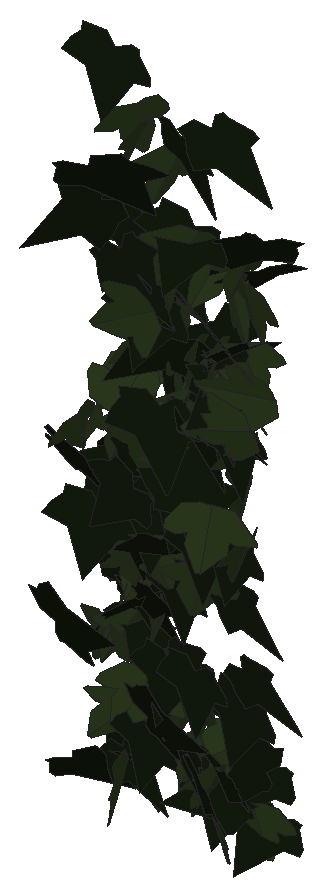
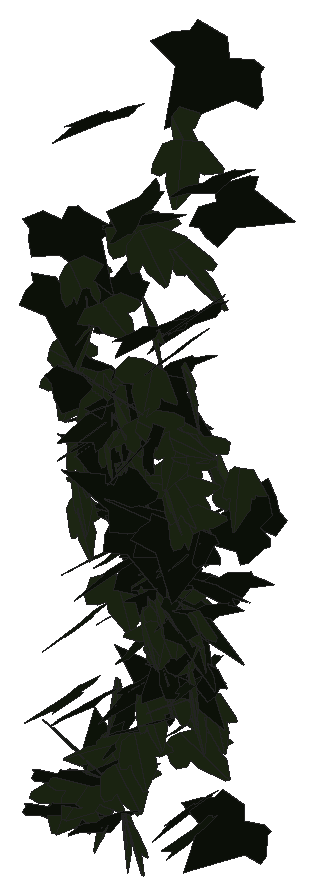
# SketchUp Ruby script. Lengths in inches.
U = 1.inch
M = Sketchup.active_model
def pt(a) = Geom::Point3d.new(a.map { |v| v * U })
def face(e, loops, mat)
  f = e.add_face(loops[0].map { |a| pt(a) })
  loops[1..].each { |l| e.add_face(l.map { |a| pt(a) }).erase! }
  f.material = f.back_material = mat if mat
  f
end
# faces: each face lists its corners as indices into pts; further lists are holes
def faces(e, pts, list, mat = nil) = list.each { |f| face(e, (f[0].is_a?(Array) ? f : [f]).map { |l| l.map { |i| pts[i] } }, mat) }
# xy, xz, yz: faces in a plane at the given z, y or x. An outline is a flat list of corners, or four numbers for a rectangle; further outlines are holes
def ring(l) = l.size == 4 ? [[l[0], l[1]], [l[2], l[1]], [l[2], l[3]], [l[0], l[3]]] : l.each_slice(2).to_a
def flat(e, list, mat, &to3) = list.each { |f| face(e, (f[0].is_a?(Array) ? f : [f]).map { |l| ring(l).map { |u, v| to3.(u, v) } }, mat) }
def xy(e, z, list, mat = nil) = flat(e, list, mat) { |x, y| [x, y, z] }
def xz(e, y, list, mat = nil) = flat(e, list, mat) { |x, z| [x, y, z] }
def yz(e, x, list, mat = nil) = flat(e, list, mat) { |y, z| [x, y, z] }
def lines(e, pts, list) = list.each { |a, b| e.add_line(pt(pts[a]), pt(pts[b])) }
# prism: a flat outline (further loops are holes) pulled along v
def prism(e, loops, v, mat = nil)
  f = face(e, loops, mat); d = Geom::Vector3d.new(v.map { |x| x * U })
  f.pushpull(f.normal.samedirection?(d) ? d.length : -d.length)
end
def box(e, o, s, mat = nil) = prism(e, [[o, [o[0] + s[0], o[1], o[2]], [o[0] + s[0], o[1] + s[1], o[2]], [o[0], o[1] + s[1], o[2]]]], [0, 0, s[2]], mat)
def at(x, y, z, deg = 0) = Geom::Transformation.translation(pt([x, y, z])) * Geom::Transformation.rotation(ORIGIN, Z_AXIS, deg.degrees)
def axes(o, x, y, z) = Geom::Transformation.new([*x, 0, *y, 0, *z, 0, *pt(o).to_a, 1])
def part(name) = M.definitions.add(name)
# library, detail: a bought-in or finely detailed component or shape, given as its bounding box
def library(name, o, s) = part(name).tap { |d| box(d.entities, o, s) }
def detail(e, o, s) = box(e.add_group.entities, o, s)
def put(e, d, t, mat = nil) = e.add_instance(d, t).tap { |i| i.material = mat if mat }
def group(e, t, mat = nil) = e.add_group.tap { |g| g.transformation = t; g.material = mat if mat }.entities
root = M.entities
M.materials.add("1026 AP 7946 SUNNY SIDE UP").color = [254, 231, 186]
M.materials.add("efeu1").color = [18, 25, 13]
M.materials.add("efeu2").color = [43, 57, 29]
c1 = part("ivyleaf_10")
p = [[0,0.5,-0.03],[-0.0625,2.02,-0.43],[-0.19,2.01,-0.46],[-0.54,1.05,-0.29],[-0.52,0.625,-0.18],[-0.83,0.76,-0.28],
  [-1.16,0.64,-0.33],[-1.15,0.33,-0.24],[-0.77,-0.39,0.02],[-0.3,-0.51,0.16],[0.04,-0.48,0.23],[-0.02,2.01,-0.4375],
  [-0.06,2.01,-0.43],[0.04,-0.49,0.23],[0.67,-0.49,0.14],[1.38,0.36,-0.2],[1.375,0.51,-0.24],[0.81,0.65,-0.19],
  [0.62,0.59,-0.15],[0.6,1.09,-0.28],[0.5,1.23,-0.31]]
faces(c1.entities,p,[[0,1,2,3,4,5,6,7,8,9,10],[11,12,0,13,14,15,16,17,18,19,20]],"efeu2")
c2 = part("ivyleaf_9")
p = [[1.54,2.16,1.25],[1.36,2.04,1.19],[-0.21,0.99,0.68],[-0.71,1.11,0.82],[-0.85,0.86,0.67],[-0.8,0.17,0.21],
  [-0.9,-0.01,0.1],[-0.67,-0.16,-0.02],[-0.08,-0.08,-0.05],[-0.03,-0.6,-0.4],[0.65,-0.88,-0.66],[0.83,-0.6,-0.49],
  [1.29,-0.42,-0.43],[1.8125,-0.07,-0.26],[1.21,0.44,0.15]]
faces(c2.entities,p,[[0,1,2,3,4,5,6,7,8,9,10,11,12,13,14]],"efeu1")
put(root,c1,axes([110.04,212.36,281.81],[-0.41666,0.10734,0.14692],[-0.23087,0.01217,-0.29167],[-0.15825,-0.30039,0.0387]),"1026 AP 7946 SUNNY SIDE UP")
put(root,c2,axes([109.94,212.88,284.09],[-0.47214,-0.12626,-0.0508],[0.11412,-0.05049,-0.32712],[0.17953,-0.29995,0.07433]),"1026 AP 7946 SUNNY SIDE UP")
put(root,c1,axes([109.9,211.86,285.31],[-0.0792,-0.30831,-0.14412],[0.04397,0.13539,-0.321],[0.52941,-0.05737,0.0051]),"1026 AP 7946 SUNNY SIDE UP")
put(root,c2,axes([109.79,212.8125,290.68],[-0.17446,-0.33344,0.05781],[0.00749,-0.06258,-0.36155],[0.53213,-0.10844,0.02404]),"1026 AP 7946 SUNNY SIDE UP")
put(root,c2,axes([109.52,211.96,284.73],[0.47639,-0.18609,0.10813],[0.1178,-0.07997,-0.36564],[0.31548,0.31086,-0.02674]),"1026 AP 7946 SUNNY SIDE UP")
put(root,c2,axes([109.76,212.02,279.81],[0.40702,0.22041,0.08662],[0.11869,0.03893,-0.34948],[-0.35069,0.26898,-0.01774]),"1026 AP 7946 SUNNY SIDE UP")
put(root,c2,axes([110.2,212.86,283.61],[-0.32806,0.22636,-0.11711],[0.00301,-0.14739,-0.30342],[-0.39919,-0.18714,0.09395]),"1026 AP 7946 SUNNY SIDE UP")
put(root,c1,axes([109.91,212.86,283.06],[-0.15896,0.28142,-0.13311],[0.00088,-0.13741,-0.30579],[-0.48797,-0.09192,0.04281]),"1026 AP 7946 SUNNY SIDE UP")
put(root,c1,axes([110.04,212.81,282.52],[0.1984,-0.29601,-0.13587],[-0.0281,0.13317,-0.32895],[0.50771,0.12305,0.03489]),"1026 AP 7946 SUNNY SIDE UP")
put(root,c2,axes([109.77,212.93,282.61],[0.17851,-0.30152,0.00504],[0.0021,-0.00656,-0.33195],[0.47422,0.11353,-0.00043]),"1026 AP 7946 SUNNY SIDE UP")
put(root,c2,axes([110.2,212.76,283.33],[-0.1289,0.31552,-0.02923],[0.0045,-0.03042,-0.33598],[-0.49837,-0.08188,0.00453]),"1026 AP 7946 SUNNY SIDE UP")
put(root,c1,axes([110.04,212.71,281.92],[0.11298,-0.31237,-0.0527],[0.0003,0.05068,-0.3297],[0.49726,0.07094,0.01218]),"1026 AP 7946 SUNNY SIDE UP")
put(root,c1,axes([110.1,212.8,284.97],[-0.16419,-0.30071,0.1012],[-0.01401,-0.1024,-0.3276],[0.49807,-0.10201,0.02414]),"1026 AP 7946 SUNNY SIDE UP")
put(root,c2,axes([109.92,212.86,283.61],[-0.18322,-0.30247,-0.04321],[0.05939,0.02843,-0.33278],[0.47611,-0.11995,0.02488]),"1026 AP 7946 SUNNY SIDE UP")
put(root,c1,axes([110.12,212.78,287.3],[0.23305,-0.29479,-0.1054],[-0.04314,0.09866,-0.33878],[0.4879,0.14953,0.02039]),"1026 AP 7946 SUNNY SIDE UP")
put(root,c2,axes([110.04,212.16,283.79],[-0.29842,-0.26578,-0.04943],[0.05476,0.03221,-0.33611],[0.4207,-0.19272,0.00869]),"1026 AP 7946 SUNNY SIDE UP")
put(root,c1,axes([110.05,212.02,285.23],[0.25096,-0.30946,0.13961],[-0.07581,0.12945,0.35912],[-0.5269,-0.16602,0.01483]),"1026 AP 7946 SUNNY SIDE UP")
put(root,c1,axes([110.21,212.8,285.4],[-0.15197,-0.28651,0.14751],[-0.01866,-0.14794,-0.31056],[0.50445,-0.09179,0.03295]),"1026 AP 7946 SUNNY SIDE UP")
put(root,c1,axes([110.19,212.92,283.47],[-0.51219,-0.0183,0.00928],[-0.01117,-0.03499,-0.33442],[0.03014,-0.32398,0.03367]),"1026 AP 7946 SUNNY SIDE UP")
put(root,c1,axes([110.1,212.8,282.99],[-0.42669,0.15548,-0.0781],[0.07139,-0.07375,-0.31994],[-0.26309,-0.27218,0.03985]),"1026 AP 7946 SUNNY SIDE UP")
put(root,c2,axes([110.17,212.84,284.76],[0.25049,0.28661,-0.04984],[-0.01719,-0.05107,-0.33775],[-0.45715,0.15897,-0.01461]),"1026 AP 7946 SUNNY SIDE UP")
put(root,c2,axes([109.81,212.88,282.82],[-0.03357,-0.03606,-0.33211],[0.48366,0.09971,-0.03191],[0.16098,-0.3071,0.02663]),"1026 AP 7946 SUNNY SIDE UP")
put(root,c1,axes([110.26,212.55,281.96],[-0.11931,-0.26401,0.18239],[-0.0022,-0.18325,-0.28084],[0.50114,-0.06366,0.04219]),"1026 AP 7946 SUNNY SIDE UP")
put(root,c2,axes([110.01,212.79,279.85],[0.1687,-0.29382,0.00052],[0.00743,-0.00059,-0.32221],[0.46196,0.10731,0.00499]),"1026 AP 7946 SUNNY SIDE UP")
put(root,c1,axes([110.62,212.93,286.4],[0.12624,-0.03617,-0.33517],[-0.50533,0.05388,-0.08761],[0.09619,0.33054,-0.02039]),"1026 AP 7946 SUNNY SIDE UP")
put(root,c1,axes([110.22,212.875,283.46],[-0.46451,0.1121,-0.0857],[0.07479,-0.10372,-0.31619],[-0.207,-0.28903,0.07807]),"1026 AP 7946 SUNNY SIDE UP")
put(root,c1,axes([110.1875,212.74,285.9],[0.31011,0.26192,-0.06047],[-0.02993,-0.06085,-0.33743],[-0.42151,0.19702,-0.02053]),"1026 AP 7946 SUNNY SIDE UP")
put(root,c2,axes([110.46,212.49,282.34],[-0.12383,0.26762,-0.16676],[-0.00197,-0.16874,-0.28508],[-0.49303,-0.06654,0.04302]),"1026 AP 7946 SUNNY SIDE UP")
put(root,c1,axes([110.33,212.87,283.67],[-0.11266,-0.30785,0.09073],[0.00004,-0.09203,-0.3255],[0.50424,-0.06877,0.0203]),"1026 AP 7946 SUNNY SIDE UP")
put(root,c1,axes([110.26,212.82,286.22],[-0.17743,-0.2893,-0.1302],[0.10691,0.10701,-0.31842],[0.48371,-0.12977,0.02262]),"1026 AP 7946 SUNNY SIDE UP")
put(root,c2,axes([110.12,212.59,288.3125],[0.09405,-0.34295,-0.02835],[0.00204,0.02618,-0.35843],[0.54075,0.05955,0.00628]),"1026 AP 7946 SUNNY SIDE UP")
put(root,c1,axes([110.4,212.92,283.68],[0.02679,-0.30085,0.12778],[0.01035,-0.12557,-0.31116],[0.51261,0.01826,-0.0004]),"1026 AP 7946 SUNNY SIDE UP")
put(root,c2,axes([110.11,212.85,284.5],[0.2487,-0.28915,-0.0526],[0.00641,0.05831,-0.33767],[0.46122,0.15511,0.03306]),"1026 AP 7946 SUNNY SIDE UP")
put(root,c1,axes([110.41,212.84,285.5],[0.11571,-0.3282,-0.03082],[-0.01063,0.02723,-0.34635],[0.51784,0.07389,-0.00022]),"1026 AP 7946 SUNNY SIDE UP")
put(root,c1,axes([110.46,212.8,282.91],[-0.30233,-0.20081,0.16911],[-0.01131,-0.20138,-0.26182],[0.40881,-0.15407,0.11782]),"1026 AP 7946 SUNNY SIDE UP")
put(root,c1,axes([110.59,212.16,280.88],[-0.33477,-0.11795,0.21363],[-0.19297,-0.18518,-0.23863],[0.32275,-0.23306,0.07892]),"1026 AP 7946 SUNNY SIDE UP")
put(root,c2,axes([110.09,212.68,284.8125],[0.50903,0.02201,0.07735],[0.11601,0.01895,-0.33387],[-0.0404,0.33175,0.01589]),"1026 AP 7946 SUNNY SIDE UP")
put(root,c2,axes([110.23,212.875,283.61],[0.22883,-0.28573,-0.0673],[-0.07302,0.04771,-0.32946],[0.45448,0.15153,-0.01905]),"1026 AP 7946 SUNNY SIDE UP")
put(root,c2,axes([110.45,212.82,281.85],[-0.19306,-0.2678,0.12855],[0.02907,-0.1434,-0.29555],[0.46466,-0.1023,0.0719]),"1026 AP 7946 SUNNY SIDE UP")
put(root,c1,axes([110.44,212.88,283.1],[0.29975,0.26211,0.03925],[-0.00229,0.04616,-0.33236],[-0.41615,0.18854,0.0301]),"1026 AP 7946 SUNNY SIDE UP")
put(root,c2,axes([110.36,212.35,280.02],[0.1753,-0.25838,-0.14486],[-0.05545,0.13598,-0.28843],[0.4581,0.11533,0.02052]),"1026 AP 7946 SUNNY SIDE UP")
put(root,c1,axes([110.61,212.32,283.28],[-0.17129,-0.30335,-0.03779],[0.0265,0.03109,-0.33182],[0.47942,-0.1101,0.00484]),"1026 AP 7946 SUNNY SIDE UP")
put(root,c2,axes([110.4,212.53,282.5],[0.49764,-0.03435,-0.06061],[-0.09767,-0.03285,-0.32571],[0.04336,0.32019,-0.038]),"1026 AP 7946 SUNNY SIDE UP")
put(root,c2,axes([110.47,212.73,287.57],[-0.05599,-0.31485,0.14173],[-0.02965,-0.13811,-0.32722],[0.54059,-0.04018,-0.00327]),"1026 AP 7946 SUNNY SIDE UP")
put(root,c1,axes([110.66,212.43,284.99],[-0.52543,0.01637,0.01731],[-0.02862,-0.03164,-0.34322],[-0.0231,-0.33308,0.03149]),"1026 AP 7946 SUNNY SIDE UP")
put(root,c2,axes([110.77,211.24,289.31],[-0.05967,-0.02786,-0.39694],[0.10582,-0.38156,0.01937],[-0.5979,-0.06475,0.04304]),"1026 AP 7946 SUNNY SIDE UP")
put(root,c2,axes([110.54,212.69,283.85],[-0.17492,-0.30837,-0.03718],[0.04587,0.02592,-0.33703],[0.48572,-0.1135,0.01844]),"1026 AP 7946 SUNNY SIDE UP")
put(root,c2,axes([110.46,212.87,283.74],[-0.05275,-0.30804,-0.11488],[0.08443,0.10366,-0.31598],[0.50722,-0.04929,0.04065]),"1026 AP 7946 SUNNY SIDE UP")
put(root,c2,axes([110.69,212.06,284.39],[-0.22147,-0.2116,0.21977],[-0.0842,-0.21547,-0.25642],[0.46627,-0.13942,0.05809]),"1026 AP 7946 SUNNY SIDE UP")
put(root,c1,axes([110.72,212.95,283.2],[0.07818,-0.31666,-0.04946],[-0.00094,0.04667,-0.32988],[0.5032,0.04929,0.00707]),"1026 AP 7946 SUNNY SIDE UP")
put(root,c2,axes([110.85,212.88,285.98],[0.01886,-0.12095,0.32264],[-0.04553,0.31253,0.12703],[-0.52694,-0.03134,0.00057]),"1026 AP 7946 SUNNY SIDE UP")
put(root,c2,axes([110.47,212.17,288],[0.1312,-0.29596,-0.19423],[-0.02416,0.18881,-0.31405],[0.54984,0.07892,0.03255]),"1026 AP 7946 SUNNY SIDE UP")
put(root,c1,axes([110.54,212.0625,285.73],[0.505,0.12235,-0.16015],[0.16605,0.1461,0.34254],[0.26405,-0.32586,0.09089]),"1026 AP 7946 SUNNY SIDE UP")
put(root,c1,axes([110.8,212.55,282.24],[0.17532,-0.2647,-0.15298],[-0.08397,0.137,-0.29507],[0.46862,0.12358,0.00436]),"1026 AP 7946 SUNNY SIDE UP")
put(root,c1,axes([110.61,212.95,283.48],[0.42521,-0.15269,0.09682],[0.11307,-0.06515,-0.31961],[0.25904,0.27907,-0.01943]),"1026 AP 7946 SUNNY SIDE UP")
put(root,c1,axes([110.79,212.87,287.19],[-0.5112,0.09624,0.01092],[-0.02827,-0.02546,-0.34811],[-0.1495,-0.32426,0.0285]),"1026 AP 7946 SUNNY SIDE UP")
put(root,c1,axes([110.83,212.84,289.32],[-0.17502,-0.31063,0.11971],[-0.00115,-0.12418,-0.3383],[0.52246,-0.10433,0.03936]),"1026 AP 7946 SUNNY SIDE UP")
put(root,c2,axes([110.93,212.86,284.63],[0.06964,0.29132,-0.15645],[-0.02346,-0.15297,-0.30436],[-0.51725,0.04616,-0.00726]),"1026 AP 7946 SUNNY SIDE UP")
put(root,c1,axes([110.83,212.03,290.43],[-0.25565,-0.33335,-0.08787],[0.07636,0.06905,-0.38144],[0.53489,-0.16918,0.01246]),"1026 AP 7946 SUNNY SIDE UP")
put(root,c2,axes([110.77,212.49,287.14],[-0.21482,-0.30826,0.07268],[-0.01923,-0.07354,-0.34728],[0.49749,-0.13595,0.01796]),"1026 AP 7946 SUNNY SIDE UP")
put(root,c1,axes([110.81,212.35,283.42],[-0.44558,-0.14871,-0.08246],[0.14181,-0.00298,-0.32668],[0.22377,-0.29422,0.04282]),"1026 AP 7946 SUNNY SIDE UP")
put(root,c1,axes([110.92,212.68,281.61],[-0.02839,-0.32295,0.02154],[0.00029,-0.02279,-0.33335],[0.50907,-0.018,0.00139]),"1026 AP 7946 SUNNY SIDE UP")
put(root,c2,axes([111.11,212.49,286.68],[0.02936,0.09354,-0.34254],[-0.12491,-0.32345,-0.10007],[-0.52939,0.08151,0.00461]),"1026 AP 7946 SUNNY SIDE UP")
put(root,c2,axes([111.06,212.26,283.61],[0.17392,0.28189,-0.15822],[-0.07174,-0.1487,-0.31264],[-0.50087,0.11918,-0.01016]),"1026 AP 7946 SUNNY SIDE UP")
put(root,c1,axes([111,211.98,281.47],[0.52597,0.0736,-0.11388],[-0.15666,-0.0607,-0.35124],[-0.13891,0.34716,-0.03508]),"1026 AP 7946 SUNNY SIDE UP")
put(root,c2,axes([110.75,212.75,287.92],[0.04706,-0.31716,-0.14479],[0.05467,0.14132,-0.32423],[0.54159,0.0133,0.04531]),"1026 AP 7946 SUNNY SIDE UP")
put(root,c1,axes([111.01,212.96,279.65],[0.30283,-0.23732,-0.04399],[-0.00947,0.04819,-0.31349],[0.37866,0.191,0.02734]),"1026 AP 7946 SUNNY SIDE UP")
put(root,c2,axes([110.98,213,284.97],[-0.38679,-0.19645,-0.10247],[0.16895,0.02121,-0.32036],[0.30131,-0.26407,0.04809]),"1026 AP 7946 SUNNY SIDE UP")
put(root,c2,axes([110.87,212.9,285.99],[0.20658,-0.29115,-0.11068],[-0.10296,0.08621,-0.3277],[0.47608,0.14498,-0.02284]),"1026 AP 7946 SUNNY SIDE UP")
put(root,c1,axes([111.02,212.84,286.29],[0.07666,0.31882,-0.10109],[-0.05894,-0.09514,-0.33207],[-0.52204,0.05756,0.02265]),"1026 AP 7946 SUNNY SIDE UP")
put(root,c2,axes([111.01,212.94,281.33],[-0.22303,-0.26383,0.10753],[0.01523,-0.12274,-0.30244],[0.44675,-0.12753,0.06399]),"1026 AP 7946 SUNNY SIDE UP")
put(root,c1,axes([111.12,212.68,280.89],[-0.14606,-0.30173,0.00557],[0.01114,-0.00963,-0.32514],[0.47444,-0.09266,0.00935]),"1026 AP 7946 SUNNY SIDE UP")
put(root,c2,axes([110.92,212.82,282.67],[-0.00412,-0.29575,0.13411],[0.02551,-0.13182,-0.30503],[0.50853,0.00422,0.01639]),"1026 AP 7946 SUNNY SIDE UP")
put(root,c1,axes([111.16,212.92,279.67],[0.13285,-0.27646,-0.11543],[0.00095,0.115,-0.29531],[0.46813,0.07822,0.03336]),"1026 AP 7946 SUNNY SIDE UP")
put(root,c1,axes([111.18,212.35,287.8],[0.29125,-0.28309,-0.08825],[-0.03686,0.08481,-0.34699],[0.46287,0.18488,0.02789]),"1026 AP 7946 SUNNY SIDE UP")
put(root,c2,axes([110.97,212.8,284.96],[0.15429,0.29054,-0.13288],[0.05794,0.12542,0.31661],[0.49753,-0.10471,0.00434]),"1026 AP 7946 SUNNY SIDE UP")
put(root,c2,axes([111.13,211.92,280.74],[-0.08525,-0.29,0.14491],[-0.0065,-0.14366,-0.30407],[0.5079,-0.05051,0.02043]),"1026 AP 7946 SUNNY SIDE UP")
put(root,c1,axes([111.26,211.54,290.49],[0.12831,-0.33596,0.10108],[0.03,-0.09829,-0.35672],[0.55037,0.08368,-0.00412]),"1026 AP 7946 SUNNY SIDE UP")
put(root,c1,axes([111.37,212.33,285.02],[-0.20512,-0.28387,0.11099],[-0.03528,-0.10968,-0.32153],[0.47703,-0.13018,0.02394]),"1026 AP 7946 SUNNY SIDE UP")
put(root,c1,axes([111.3125,212.28,281.375],[0.06316,-0.30272,0.09418],[0.02887,-0.0915,-0.31507],[0.49718,0.04377,0.00633]),"1026 AP 7946 SUNNY SIDE UP")
put(root,c2,axes([111.02,212.78,289.69],[0.18683,-0.32958,0.13084],[0.05591,-0.12414,-0.36156],[0.55364,0.12376,-0.00764]),"1026 AP 7946 SUNNY SIDE UP")
put(root,c2,axes([111.17,212.09,285.8],[-0.16122,-0.36141,-0.0643],[0.0645,0.05096,-0.38584],[0.57252,-0.10751,0.02537]),"1026 AP 7946 SUNNY SIDE UP")
put(root,c1,axes([111.4,212.72,280.3125],[-0.22353,-0.25621,0.11746],[-0.01996,-0.12342,-0.29893],[0.44144,-0.13531,0.04596]),"1026 AP 7946 SUNNY SIDE UP")
put(root,c1,axes([111.28,212.87,286.51],[0.13537,-0.29309,0.14519],[0.09749,-0.13008,-0.31474],[0.50316,0.10405,0.02192]),"1026 AP 7946 SUNNY SIDE UP")
put(root,c1,axes([111.44,212.65,285.77],[-0.27411,-0.26224,0.11837],[-0.02814,-0.12599,-0.32078],[0.45026,-0.16752,0.05202]),"1026 AP 7946 SUNNY SIDE UP")
put(root,c2,axes([111.35,212.52,284.48],[-0.42264,-0.15014,-0.13133],[0.1877,0.04555,-0.31642],[0.24524,-0.29361,0.01586]),"1026 AP 7946 SUNNY SIDE UP")
put(root,c2,axes([111.17,212.33,281.76],[0.1457,-0.2171,-0.23601],[-0.04767,0.23027,-0.23738],[0.49258,0.0865,0.04684]),"1026 AP 7946 SUNNY SIDE UP")
put(root,c2,axes([111.28,212.17,281.72],[-0.10456,-0.2876,0.13693],[-0.02091,-0.13482,-0.30445],[0.49883,-0.06593,0.01594]),"1026 AP 7946 SUNNY SIDE UP")
put(root,c1,axes([111.42,212.76,286.125],[0.09943,-0.3349,-0.01855],[0.03058,0.02002,-0.3502],[0.52632,0.0621,0.02385]),"1026 AP 7946 SUNNY SIDE UP")
put(root,c1,axes([111.72,210.95,288.02],[0.37388,-0.14777,-0.28081],[-0.37353,0.13228,-0.28747],[0.31151,0.33598,-0.00767]),"1026 AP 7946 SUNNY SIDE UP")
put(root,c2,axes([111.06,209.99,283.33],[0.07703,-0.08837,0.39051],[0.32588,-0.31807,-0.10571],[0.51897,0.21285,0.00841]),"1026 AP 7946 SUNNY SIDE UP")
put(root,c2,axes([111.27,212.66,283.89],[0.23626,-0.21641,-0.21497],[-0.07322,0.21238,-0.26175],[0.46564,0.1432,0.06791]),"1026 AP 7946 SUNNY SIDE UP")
put(root,c1,axes([111.56,212.69,285.62],[0.06744,-0.33524,0.0203],[0.004,-0.02146,-0.3483],[0.52821,0.04297,0.00004]),"1026 AP 7946 SUNNY SIDE UP")
put(root,c1,axes([111.37,210.98,280.65],[0.16006,-0.19305,0.32232],[0.26132,-0.26669,-0.226],[0.51729,0.19446,0.01444]),"1026 AP 7946 SUNNY SIDE UP")
put(root,c2,axes([111.94,212.875,286.78],[-0.36911,0.20931,0.13194],[-0.24318,0.00942,-0.31073],[-0.29831,-0.26667,0.09005]),"1026 AP 7946 SUNNY SIDE UP")
put(root,c1,axes([111.61,212.79,287.95],[0.26706,0.24758,-0.16732],[-0.1788,-0.12009,-0.30912],[-0.43121,0.20313,0.02455]),"1026 AP 7946 SUNNY SIDE UP")
put(root,c1,axes([111.7,212.43,283.19],[-0.44566,-0.14546,0.07633],[-0.07782,-0.06662,-0.32651],[0.24522,-0.28549,0.0351]),"1026 AP 7946 SUNNY SIDE UP")
put(root,c2,axes([111.39,212.55,285.57],[0.19152,-0.3133,0.05267],[0.00817,-0.05469,-0.34628],[0.49955,0.12101,-0.01453]),"1026 AP 7946 SUNNY SIDE UP")
put(root,c2,axes([111.42,212.21,280.66],[0.14807,-0.28591,0.12843],[0.02948,-0.12649,-0.31016],[0.49058,0.0939,-0.02012]),"1026 AP 7946 SUNNY SIDE UP")
put(root,c2,axes([111.62,212.97,279.59],[-0.16265,-0.28629,0.04824],[0.00135,-0.05174,-0.31334],[0.45656,-0.10184,0.01811]),"1026 AP 7946 SUNNY SIDE UP")
put(root,c2,axes([111.3,211.72,281.13],[0.14973,-0.11356,0.35167],[0.28627,-0.29012,-0.15316],[0.48901,0.20461,-0.01802]),"1026 AP 7946 SUNNY SIDE UP")
put(root,c2,axes([111.45,212.93,286.29],[0.39825,-0.2232,-0.00703],[-0.02958,-0.01296,-0.34711],[0.34982,0.253,-0.02135]),"1026 AP 7946 SUNNY SIDE UP")
put(root,c1,axes([111.88,211.88,288.81],[-0.27488,-0.2895,0.17147],[-0.08481,-0.16279,-0.34758],[0.5195,-0.17976,0.03399]),"1026 AP 7946 SUNNY SIDE UP")
put(root,c2,axes([111.85,212,284.63],[-0.51579,0.03787,0.11664],[0.1821,0.02303,0.33848],[0.04432,0.34618,-0.03322]),"1026 AP 7946 SUNNY SIDE UP")
put(root,c1,axes([111.78,212.86,286.57],[0.07066,0.22999,-0.25245],[-0.11689,-0.23565,-0.24199],[-0.5169,0.08473,0.02021]),"1026 AP 7946 SUNNY SIDE UP")
put(root,c2,axes([111.62,212.87,285.89],[0.0391,-0.33113,0.05738],[0.00293,-0.0576,-0.34241],[0.52847,0.02482,-0.00235]),"1026 AP 7946 SUNNY SIDE UP")
put(root,c2,axes([111.4375,212.89,285.53],[0.24804,-0.1805,0.24112],[0.20443,-0.19717,-0.24699],[0.4188,0.20315,-0.02224]),"1026 AP 7946 SUNNY SIDE UP")
put(root,c2,axes([111.65,212.37,283.77],[-0.032,-0.30641,0.11855],[0.03013,-0.11795,-0.31599],[0.51475,-0.01215,0.02586]),"1026 AP 7946 SUNNY SIDE UP")
put(root,c2,axes([111.66,212.86,286.04],[0.02283,-0.33181,0.06291],[-0.00146,-0.06304,-0.3425],[0.53104,0.01409,-0.00365]),"1026 AP 7946 SUNNY SIDE UP")
put(root,c2,axes([111.84,211.97,288.93],[-0.27939,-0.3001,0.05996],[-0.01545,-0.06364,-0.35883],[0.48094,-0.17638,0.02331]),"1026 AP 7946 SUNNY SIDE UP")
put(root,c1,axes([111.86,212.25,281.35],[0.14331,-0.24922,-0.18585],[0.04598,0.19292,-0.26026],[0.48027,0.0559,0.08038]),"1026 AP 7946 SUNNY SIDE UP")
put(root,c1,axes([111.87,212.46,279.41],[-0.25295,0.2719,0.0187],[-0.01952,0.01195,-0.32536],[-0.42789,-0.16128,0.00379]),"1026 AP 7946 SUNNY SIDE UP")
put(root,c2,axes([111.71,209.93,290.76],[0.54604,0.25505,0.02975],[0.06581,-0.01079,-0.44261],[-0.39796,0.34818,-0.03237]),"1026 AP 7946 SUNNY SIDE UP")
put(root,c2,axes([112.11,212.85,286.74],[-0.12279,0.24161,-0.23252],[-0.02211,-0.2355,-0.25452],[-0.52089,-0.04696,0.06562]),"1026 AP 7946 SUNNY SIDE UP")
put(root,c1,axes([111.9,212.875,287.48],[-0.0912,0.33585,-0.01025],[-0.02196,-0.01443,-0.3508],[-0.52797,-0.05742,0.01636]),"1026 AP 7946 SUNNY SIDE UP")
put(root,c2,axes([112.01,212.72,286.06],[-0.28865,-0.20153,0.20492],[-0.09261,-0.20602,-0.27068],[0.4368,-0.17685,0.07803]),"1026 AP 7946 SUNNY SIDE UP")
put(root,c2,axes([112.2,212.49,279.84],[-0.25496,-0.08533,0.2866],[-0.29885,-0.21082,-0.18165],[0.34744,-0.24395,0.05406]),"1026 AP 7946 SUNNY SIDE UP")
put(root,c1,axes([112.07,212.14,280.31],[-0.01695,-0.30648,0.09304],[0.00079,-0.09213,-0.31645],[0.50318,-0.01018,0.00363]),"1026 AP 7946 SUNNY SIDE UP")
put(root,c1,axes([111.88,212.47,280.48],[0.12617,-0.01949,-0.32732],[0.22649,0.2943,0.0206],[0.44616,-0.14389,0.08211]),"1026 AP 7946 SUNNY SIDE UP")
put(root,c1,axes([111.97,212.77,279.99],[-0.42973,-0.1231,-0.10992],[0.17819,0.00416,-0.30596],[0.18301,-0.2931,0.0398]),"1026 AP 7946 SUNNY SIDE UP")
put(root,c2,axes([111.96,212.72,283.66],[-0.11121,-0.29686,0.1232],[0.02052,-0.12675,-0.31253],[0.50381,-0.06037,0.03992]),"1026 AP 7946 SUNNY SIDE UP")
put(root,c2,axes([111.89,212.78,282.8],[0.25174,-0.23988,-0.14809],[-0.06203,0.14306,-0.29313],[0.43422,0.1595,0.04398]),"1026 AP 7946 SUNNY SIDE UP")
put(root,c1,axes([112.06,212.85,286.66],[-0.41105,-0.20419,-0.08088],[0.15689,-0.00438,-0.3355],[0.30539,-0.27258,0.06349]),"1026 AP 7946 SUNNY SIDE UP")
put(root,c2,axes([112.26,212.89,288],[0.14945,0.32744,-0.03781],[-0.08456,-0.0242,-0.34837],[-0.51149,0.09968,0.04655]),"1026 AP 7946 SUNNY SIDE UP")
put(root,c1,axes([112.2,212.75,288.28],[-0.08723,-0.33314,0.08732],[-0.002,-0.08757,-0.34819],[0.54126,-0.05402,0.01279]),"1026 AP 7946 SUNNY SIDE UP")
put(root,c1,axes([112.56,212.08,285.95],[-0.23193,0.02061,0.33353],[-0.49721,-0.08803,-0.1432],[0.11314,-0.3446,0.05438]),"1026 AP 7946 SUNNY SIDE UP")
put(root,c2,axes([112.05,212.62,285.56],[-0.01162,-0.33371,0.02831],[0.00026,-0.02938,-0.34405],[0.52676,-0.00734,0.00079]),"1026 AP 7946 SUNNY SIDE UP")
put(root,c1,axes([112.25,212.57,285.35],[-0.06279,-0.33655,-0.02845],[0.01824,0.0245,-0.34889],[0.53042,-0.04068,0.00863]),"1026 AP 7946 SUNNY SIDE UP")
put(root,c2,axes([112.14,212.77,281.18],[-0.12663,-0.30929,0.13365],[-0.02456,-0.13162,-0.32957],[0.52788,-0.08032,0.01673]),"1026 AP 7946 SUNNY SIDE UP")
put(root,c2,axes([112.32,212.99,280.125],[-0.40049,-0.17738,-0.00125],[0.02035,-0.01822,-0.31903],[0.27817,-0.25405,0.02153]),"1026 AP 7946 SUNNY SIDE UP")
put(root,c2,axes([112.01,212.9375,281.56],[0.27254,-0.23645,-0.12456],[-0.02249,0.13432,-0.29422],[0.41602,0.16216,0.06569]),"1026 AP 7946 SUNNY SIDE UP")
put(root,c1,axes([112.2,211.89,284.51],[0.53188,0.13844,-0.02513],[-0.01863,-0.0373,-0.37548],[-0.22047,0.33713,-0.0289]),"1026 AP 7946 SUNNY SIDE UP")
put(root,c1,axes([112.32,212.52,284.67],[0.06481,-0.33225,-0.04575],[0.01901,0.04429,-0.34419],[0.52635,0.03931,0.01806]),"1026 AP 7946 SUNNY SIDE UP")
put(root,c2,axes([111.9,212.02,287.57],[0.26082,-0.26917,0.22834],[0.18599,-0.18925,-0.32683],[0.51739,0.20373,0.00238]),"1026 AP 7946 SUNNY SIDE UP")
put(root,c2,axes([112.14,212.35,280.25],[-0.06955,-0.16032,0.27713],[0.0857,-0.27237,-0.15905],[0.48614,0.02508,0.06768]),"1026 AP 7946 SUNNY SIDE UP")
put(root,c1,axes([112.35,212.64,287.79],[-0.43992,0.20433,-0.00506],[-0.01631,-0.02447,-0.35605],[-0.32101,-0.27877,0.02502]),"1026 AP 7946 SUNNY SIDE UP")
put(root,c2,axes([112.69,212.49,280.42],[-0.33661,0.21384,0.11061],[-0.15212,0.05265,-0.30994],[-0.34319,-0.23308,0.02889]),"1026 AP 7946 SUNNY SIDE UP")
put(root,c2,axes([112.25,211.53,282.26],[-0.05787,-0.31123,0.09101],[0.02078,-0.09205,-0.32252],[0.50905,-0.03162,0.02351]),"1026 AP 7946 SUNNY SIDE UP")
put(root,c2,axes([112.21,211.71,280.39],[0.00854,-0.14345,0.29458],[0.03963,-0.28572,-0.14941],[0.50261,0.02497,0.00678]),"1026 AP 7946 SUNNY SIDE UP")
put(root,c1,axes([112.8,212.22,286.5],[0.13966,-0.02728,-0.34569],[-0.51364,0.07635,-0.09507],[0.12713,0.33846,-0.00432]),"1026 AP 7946 SUNNY SIDE UP")
put(root,c1,axes([112.4,212.71,279.58],[-0.48797,-0.02742,-0.05686],[0.09414,-0.07031,-0.31214],[0.022,-0.30723,0.0746]),"1026 AP 7946 SUNNY SIDE UP")
put(root,c2,axes([112.7,212.42,288.82],[0.03646,0.25549,-0.24009],[-0.156,-0.22032,-0.25868],[-0.52251,0.0836,0.06048]),"1026 AP 7946 SUNNY SIDE UP")
put(root,c1,axes([112.54,212.27,284.07],[0.00844,-0.33713,-0.01695],[-0.0145,0.01439,-0.34715],[0.5304,0.00576,-0.00922]),"1026 AP 7946 SUNNY SIDE UP")
put(root,c2,axes([112.22,211.99,290.59],[0.13473,-0.30526,-0.17427],[0.06953,0.18057,-0.31479],[0.54302,0.05262,0.08354]),"1026 AP 7946 SUNNY SIDE UP")
put(root,c2,axes([112.56,212.87,279.44],[-0.38399,-0.19045,0.0049],[0.01983,-0.02563,-0.31788],[0.29894,-0.24293,0.02739]),"1026 AP 7946 SUNNY SIDE UP")
